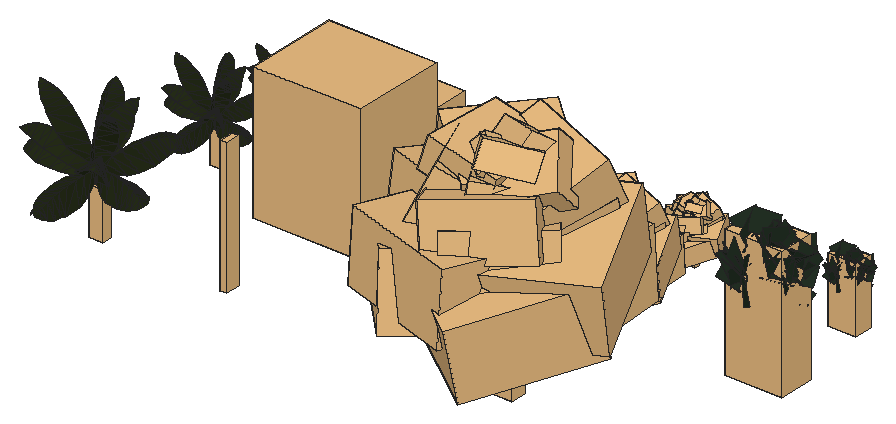
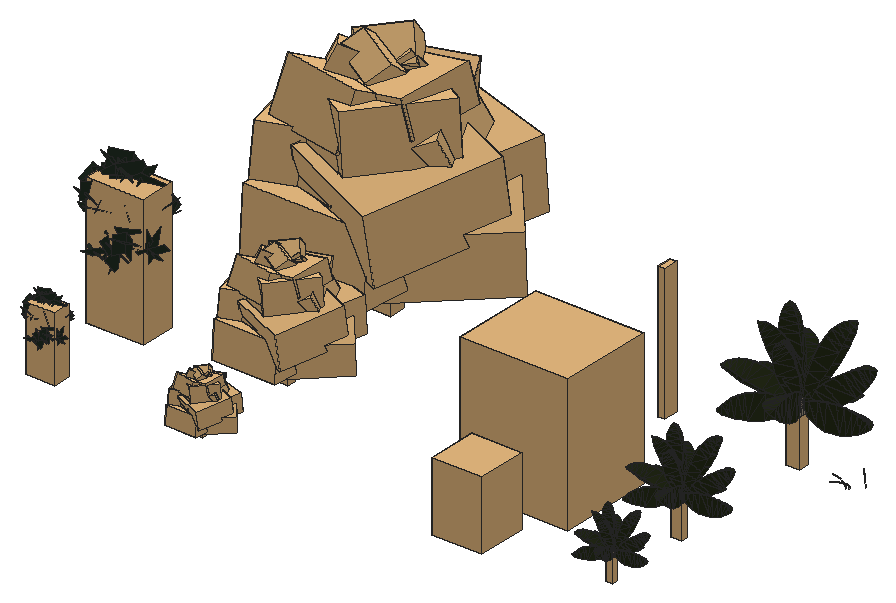
# SketchUp Ruby script. Lengths in inches.
U = 1.inch
M = Sketchup.active_model
def pt(a) = Geom::Point3d.new(a.map { |v| v * U })
def face(e, loops, mat)
  f = e.add_face(loops[0].map { |a| pt(a) })
  loops[1..].each { |l| e.add_face(l.map { |a| pt(a) }).erase! }
  f.material = f.back_material = mat if mat
  f
end
# faces: each face lists its corners as indices into pts; further lists are holes
def faces(e, pts, list, mat = nil) = list.each { |f| face(e, (f[0].is_a?(Array) ? f : [f]).map { |l| l.map { |i| pts[i] } }, mat) }
# xy, xz, yz: faces in a plane at the given z, y or x. An outline is a flat list of corners, or four numbers for a rectangle; further outlines are holes
def ring(l) = l.size == 4 ? [[l[0], l[1]], [l[2], l[1]], [l[2], l[3]], [l[0], l[3]]] : l.each_slice(2).to_a
def flat(e, list, mat, &to3) = list.each { |f| face(e, (f[0].is_a?(Array) ? f : [f]).map { |l| ring(l).map { |u, v| to3.(u, v) } }, mat) }
def xy(e, z, list, mat = nil) = flat(e, list, mat) { |x, y| [x, y, z] }
def xz(e, y, list, mat = nil) = flat(e, list, mat) { |x, z| [x, y, z] }
def yz(e, x, list, mat = nil) = flat(e, list, mat) { |y, z| [x, y, z] }
def lines(e, pts, list) = list.each { |a, b| e.add_line(pt(pts[a]), pt(pts[b])) }
# prism: a flat outline (further loops are holes) pulled along v
def prism(e, loops, v, mat = nil)
  f = face(e, loops, mat); d = Geom::Vector3d.new(v.map { |x| x * U })
  f.pushpull(f.normal.samedirection?(d) ? d.length : -d.length)
end
def box(e, o, s, mat = nil) = prism(e, [[o, [o[0] + s[0], o[1], o[2]], [o[0] + s[0], o[1] + s[1], o[2]], [o[0], o[1] + s[1], o[2]]]], [0, 0, s[2]], mat)
def at(x, y, z, deg = 0) = Geom::Transformation.translation(pt([x, y, z])) * Geom::Transformation.rotation(ORIGIN, Z_AXIS, deg.degrees)
def axes(o, x, y, z) = Geom::Transformation.new([*x, 0, *y, 0, *z, 0, *pt(o).to_a, 1])
def part(name) = M.definitions.add(name)
# library, detail: a bought-in or finely detailed component or shape, given as its bounding box
def library(name, o, s) = part(name).tap { |d| box(d.entities, o, s) }
def detail(e, o, s) = box(e.add_group.entities, o, s)
def put(e, d, t, mat = nil) = e.add_instance(d, t).tap { |i| i.material = mat if mat }
def group(e, t, mat = nil) = e.add_group.tap { |g| g.transformation = t; g.material = mat if mat }.entities
root = M.entities
M.materials.add("cocoanut_mat").color = [137, 122, 109]
M.materials.add("cocoanut_scrub").color = [165, 152, 134]
M.materials.add("coconut_test3_clean").color = [38, 45, 24]
M.materials.add("euc leaf02").color = [35, 48, 36]
c1 = library("Group\#110",[0,0,0],[259.75,161.77,589.29])
c2 = part("Blue Gum")
p = [[271.53,158.18,378.25],[270.5625,158.71,380.69],[270.37,158.83,381.17],[272.73,162.06,384.51],[213.85,150.08,152.75],[212.24,149.06,149.65],
  [150.49,110.24,344.32],[151.97,108.18,342.21],[217.47,152.58,206.91],[209.32,150.04,213.6],[153.27,112.37,338.72],[213.34,156.04,223.13],
  [212.17,155.27,219.89],[213.66,148.52,337.14],[212.6875,151.94,345.88],[201.33,160.36,0],[198.82,151.26,0.01],[228.58,150.59,468.55],
  [228.91,150.53,474.28],[226.95,148.99,472.86]]
faces(c2.entities,p,[[0,1,2],[1,0,3],[3,2,1]])
lines(c2.entities,p,[[4,5],[6,7],[8,9],[10,6],[7,10],[11,12],[13,14],[15,16],[17,18],[19,17],[18,19]])
put(c2.entities,c1,axes([324.42,234.92,0.08],[-1,0,-0.00067],[0,-1,0.00003],[-0.00067,0.00003,1]))
g1 = group(c2.entities,at(392.72,299.04,214.24))
p = [[-190.24,-45.24,49.75],[-155.8,-83.51,-0.1],[-171.1,-117.4,15.86],[-186.4,-151.3,31.82],[-220.85,-113.03,81.67],[-197.84,-62.08,57.68],
  [-156.97,-85.38,90],[-134.58,-101.98,23.98],[-207.62,-132.83,7.74],[-230.01,-116.24,73.77],[-175.11,-93.05,85.97],[-155.875,-47.35,89.82],
  [-171.875,-81.0625,28.63],[-175.09,-115.85,49.06],[-178.3125,-150.63,69.48],[-162.3125,-116.92,130.67],[-157.47,-64.63,99.96],[-108.86,-93.44,91.87],
  [-142.19,-103.1875,29.18],[-207.99,-128.51,68.93],[-174.66,-118.76,131.62],[-125.2,-99.73,101.74],[-105.25,-143.93,101.02],[-118.65,-122.91,33.83],
  [-139.46,-91.34,48.24],[-160.28,-59.76,62.65],[-146.87,-80.78,129.84],[-115.59,-128.24,108.18],[-69.65,-64.39,98.91],[-102.98,-74.13,36.22],
  [-135.88,-86.79,56.09],[-168.78,-99.45,75.97],[-135.45,-89.7,138.66],[-85.99,-70.68,108.78],[-206,0,112.1],[-205.51,-55.1,41.09],
  [-219.69,-93.37,71.26],[-233.87,-131.63,101.43],[-234.36,-76.53,172.4375],[-220.18,-38.26,142.27],[-213.05,-19.01,127.09],[-58.99,-92.56,99.73],
  [-109.77,-114.37,54.1],[-132.54,-82.69,64.86],[-155.3,-51.01,75.61],[-104.53,-29.2,121.24],[-70.31,-76.82,105.07],[-84.85,-14.67,104.44],
  [-93.72,-70.0625,59.84],[-130.5,-76.32,75.5],[-167.29,-82.57,91.16],[-158.42,-27.18,135.76],[-103.12,-17.78,112.22],[-170.99,-48.24,149.78],
  [-170.5,-103.34,78.77],[-268.88,-83.39,63.75],[-269.37,-28.29,134.76],[-195.43,-43.28,146.05],[-119.44,-162.62,158.17],[-165.08,-157.98,109.24],
  [-139.69,-139.86,87.75],[-114.31,-121.74,66.26],[-68.68,-126.38,115.19],[-94.0625,-144.5,136.68],[-106.83,-153.62,147.5],[-83.43,-178.22,123.11],
  [-129.0625,-173.58,74.18],[-150.32,-106.13,101.32],[-104.69,-110.78,150.25],[-88.71,-161.47,129.85],[-153.18,-33.52,154.23],[-187.55,-61.6,76.08],
  [-205.14,-103.18,99.27],[-222.72,-144.75,122.47],[-188.35,-116.67,200.62],[-170.77,-75.09,177.42],[-161.92,-54.17,165.75],[-126.95,-97.9375,165.85],
  [-161.32,-126.02,87.7],[-248.95,-80.33,110.85],[-214.58,-52.25,189],[-148.72,-86.59,171.6],[-365.27,-93.53,149.96],[-339.43,-156.16,87.91],
  [-290.4375,-139.67,92.34],[-241.45,-123.17,96.77],[-267.29,-60.54,158.83],[-340.93,-85.33,152.16],[-220,-209.94,88.83],[-192.18,-284.625,134.55],
  [-202.3,-275.33,156.35],[-232.93,-247.2,222.33],[-260.75,-172.52,176.61],[-240.375,-191.23,132.72],[-392.72,-100.24,198.19],[-366.88,-162.88,136.14],
  [-328.26,-131.57,121.3],[-289.64,-100.27,106.47],[-315.48,-37.63,168.52],[-373.54,-84.69,190.82],[-327.95,-161.62,221.67],[-317.1,-180.89,132.49],
  [-328.31,-131.57,120.9375],[-339.53,-82.25,109.39],[-350.38,-62.97,198.5625],[-333.52,-137.11,215.93],[-255.83,-236.76,152.47],[-329.61,-198.39,191.52],
  [-323.5,-175.58,181.2],[-305,-106.55,149.96],[-231.21,-144.93,110.9],[-243.52,-190.85,131.6875],[-205.5,-81.8,220.89],[-197.86,-85.86,131.43],
  [-243.5,-64.11,127],[-289.13,-42.35,122.57],[-296.77,-38.29,212.03],[-251.13,-60.04,216.46],[-228.17,-70.99,218.6875],[-234.33,-241.65,142.48],
  [-225.25,-222.09,231.79],[-228.94,-197.05,226.92],[-240.1,-121.29,212.17],[-249.18,-140.85,122.86],[-241.75,-191.25,132.67],[-227.68,-15.04,215.96],
  [-220.04,-19.1,126.5],[-266.95,-109.11,127.5],[-274.59,-105.04,216.95],[-239.33,-37.4,216.21],[-312.18,-35.14,201.88],[-307.82,-106.7,144.42],
  [-256.66,-99.36,139.9],[-205.5,-92.02,135.375],[-209.86,-20.46,192.83],[-286.77,-31.49,199.63],[-224.25,-107.3,143.78],[-158.47,-57.42,184.1],
  [-153.89,-76.52,200.79],[-140.05,-134.32,251.29],[-205.83,-184.2,210.96],[-215.04,-145.75,177.37],[-371.18,-63.42,218.95],[-318.87,-74.08,144.18],
  [-278.67,-86.3125,174.61],[-238.47,-98.55,205.04],[-290.78,-87.88,279.82],[-351.21,-69.49,234.07],[-314.82,-59.28,247.3],[-323.0625,-96.32,163.62],
  [-272.16,-89.61,156.15],[-221.26,-82.9,148.67],[-213.02,-45.87,232.35],[-289.54,-55.95,243.59],[-269.6,-260.65,169.64],[-261.02,-289.45,256.47],
  [-255.15,-265.53,264.0625],[-237.36,-193.15,287.04],[-245.94,-164.36,200.22],[-257.77,-212.5,184.93],[-219.98,-94.58,184.38],[-135.38,-92.14,220.14],
  [-132.93,-117.5625,216.66],[-125.5,-194.48,206.12],[-210.1,-196.92,170.36],[-242.72,-259.5,171.19],[-311.27,-292.91,222.44],[-317.8125,-269.04,229.65],
  [-337.62,-196.84,251.48],[-269.07,-163.43,200.23],[-255.89,-211.46,185.71],[-204.01,-188.2,177.79],[-188.33,-208.64,265.98],[-194.51,-184.59,272.89],
  [-213.23,-111.83,293.8125],[-228.92,-91.39,205.62],[-216.46,-139.79,191.7],[-111.12,-172.19,178.4],[-144.16,-223.61,247],[-146.96,-202.62,261.69],
  [-155.45,-139.1,306.14],[-122.41,-87.68,237.53],[-116.76,-129.9375,207.97],[-92.3,-219.25,321.53],[-140.07,-175.86,256.125],[-105.48,-191.84,220.91],
  [-70.89,-207.83,185.69],[-23.13,-251.22,251.1],[-75.12,-227.1875,304.03],[-95.32,-86.56,260.02],[-28.15,-67.53,258.27],[-24.95,-79.6,243.18],
  [-15.25,-116.11,197.51],[-82.42,-135.13,199.26],[-88.87,-110.84,229.64],[-230.35,-182.42,199.75],[-240.26,-200.67,289.25],[-235.09,-176.09,295.07],
  [-219.44,-101.74,312.67],[-209.53,-83.5,223.17],[-219.9375,-132.96,211.46],[-140.68,-151.65,266.01],[-78.24,-142.94,332.84],[-63.08,-129.17,317.2],
  [-17.2,-87.5,269.85],[-79.64,-96.22,203.02],[-110.16,-123.93,234.52],[-181.78,-155.46,254.29],[-197.87,-106.1875,330.15],[-215.8125,-92.48,317.72],
  [-270.1,-51.01,280.11],[-254.02,-100.28,204.25],[-217.9,-127.875,229.27],[-219.05,-237.83,228.68],[-246.19,-265.11,312.11],[-270.4375,-258.25,306.72],
  [-343.82,-237.49,290.4],[-316.68,-210.21,206.96],[-267.86,-224.02,217.82],[-221.64,-245.99,220.16],[-255.74,-296.14,289.1875],[-278.74,-284.87,286.3125],
  [-348.35,-250.78,277.61],[-314.25,-200.64,208.59],[-267.95,-223.32,214.37],[-214.08,-176.63,246.6],[-287.9,-162.75,299.5],[-289.8,-138.53,290.89],
  [-295.55,-65.24,264.85],[-221.72,-79.12,211.94],[-273.56,-277.41,225.52],[-332.72,-264.05,294.53],[-330.67,-238.52,291.65],[-324.47,-161.27,282.95],
  [-265.3,-174.62,213.93],[-269.43,-226.01,219.72],[-125.42,-280.5,273.74],[-154.49,-208.42,224.74],[-56.47,-175.26,217.08],[-27.39,-247.34,266.08],
  [-101.07,-272.26,271.84],[-137.08,-126.63,220.68],[-181.31,-63.4,270.55],[-159.07,-51.25,275.29],[-91.8,-14.51,289.63],[-47.57,-77.74,239.76],
  [-92.33,-102.1875,230.22],[-238.16,-243.49,222.62],[-218.34,-248.07,312.22],[-217.08,-222.36,313.49],[-213.28,-144.56,317.34],[-233.09,-139.97,227.74],
  [-235.625,-191.73,225.18],[-96.8,-128.7,236.99],[-25.62,-162.74,224.18],[-29.7,-177.8,240.28],[-42.05,-223.37,289.02],[-113.23,-189.33,301.82],
  [-105.01,-159.01,269.41],[-190.11,-164.1875,296.41],[-166.86,-101.93,340.84],[-154.3,-94.29,323.91],[-116.3,-71.16,272.67],[-139.55,-133.41,228.25],
  [-164.83,-148.8,262.33],[-190.89,-165.45,228.74],[-213.01,-227.55,273.96],[-199.51,-220.6,290.46],[-158.68,-199.56,340.39],[-136.56,-137.46,295.18],
  [-163.73,-151.45,261.96],[-108.84,-65.86,242.35],[-143.91,-74.96,326.78],[-145.22,-100.52,323.73],[-149.17,-177.86,314.51],[-114.09,-168.76,230.08],
  [-111.47,-117.3125,236.21],[-131.79,-76.12,256.875],[-89.01,-36.19,327.71],[-66.95,-47.86,321.26],[-0.2,-83.16,301.74],[-42.99,-123.09,230.91],
  [-87.39,-99.61,243.89],[-191.96,-179.86,282.46],[-135.02,-196.07,336.18],[-121.21,-181.46,326.24],[-79.42,-137.25,296.18],[-136.36,-121.05,242.47],
  [-164.16,-150.45,262.47],[-230.13,-253.21,246.97],[-260.13,-299.04,320.74],[-267.04,-276.89,331.97],[-287.96,-209.88,365.95],[-257.97,-164.06,292.17],
  [-244.05,-208.64,269.57],[-280.97,-237.22,246.96],[-334.39,-225.07,320.72],[-316.05,-210.87,331.95],[-260.54,-167.9,365.9375],[-207.12,-180.05,292.18],
  [-123.3,-254.01,336.04],[-125.12,-228.29,247.85],[-81.63,-201.01,255.39],[-38.14,-173.74,262.92],[-36.32,-199.46,351.11],[-101.69,-240.46,339.78],
  [-68.26,-134.5,260.14],[-26.24,-201.97,251.74],[-44.5,-214.15,256.34],[-99.74,-251,270.27],[-141.76,-183.53,278.67],[-121.3,-170.4,347.79],
  [-129.86,-181.96,257.04],[-33.4,-220.07,253.73],[-24.85,-208.51,344.48],[-97.34,-179.87,346.97],[-78.09,-121.04,341.08],[-129.1,-143.71,268.11],
  [-128.64,-193.18,283.74],[-128.18,-242.65,299.36],[-77.17,-219.98,372.34],[-77.86,-145.61,348.85],[-177.42,-71.46,329.51],[-152.53,-122.65,273.39],
  [-155.7,-156.33,303.27],[-158.88,-190.01,333.16],[-183.78,-138.82,389.27],[-179,-88.19,344.35],[-150.51,-90.39,274.04],[-160.0625,-83.41,365.16],
  [-137.04,-94.48,368.65],[-67.4,-127.95,379.21],[-57.85,-134.93,288.09],[-104.18,-112.66,281.07],[-94.02,-187.3,327.96],[-81.13,-138.55,389.98],
  [-69.09,-124.83,376.95],[-32.66,-83.33,337.53],[-45.54,-132.09,275.51],[-69.78,-159.69,301.74],[-118.35,-128.14,277.49],[-134.07,-116.2,367.22],
  [-118.18,-95.9,367.54],[-70.12,-34.49,368.49],[-54.4,-46.4375,278.76],[-86.375,-87.29,278.12],[-130.67,-185.64,278.8125],[-99.69,-223.89,341.79],
  [-81.85,-210.3,341.52],[-27.87,-169.2,340.6875],[-58.85,-130.95,277.71],[-94.76,-158.29,278.26],[-124.09,-168.51,302.87],[-98.25,-187.53,376.08],
  [-77.34,-181.72,370.43],[-14.08,-164.14,353.32],[-39.93,-145.12,280.11],[-82.01,-156.82,291.49],[-222.9,-199.13,376.1],[-220.07,-149.45,341.44],
  [-227.34,-168.57,313.98],[-234.62,-187.6875,286.52],[-237.45,-237.37,321.18],[-230.17,-218.25,348.64],[-226.51,-208.63,362.46],[-66.91,-203,314.13],
  [-2.98,-185.26,358.72],[-4.41,-163.74,352.56],[-8.73,-98.64,333.94],[-72.66,-116.39,289.35],[-169.41,-164.76,388.4],[-177.97,-176.3125,297.65],
  [-129.74,-195.37,296],[-81.52,-214.43,294.34],[-72.96,-202.87,385.09],[-145.46,-174.22,387.58],[-154.72,-129.21,384.88],[-129.15,-146.67,298.38],
  [-129.71,-197.46,308.96],[-130.27,-248.25,319.53],[-155.84,-230.78,406.04],[-155,-154.4375,390.14],[-202.43,-168.15,321.54],[-179.78,-204.63,388.96],
  [-158.3,-199.98,384.5],[-93.32,-185.9,371.01],[-115.96,-149.42,303.58],[-159.19,-158.79,312.5625],[-197.46,-225.01,341.1],[-194.63,-175.33,306.4375],
  [-260.05,-161.8125,321.53],[-262.88,-211.49,356.1875],[-213.71,-221.65,344.85],[-157.48,-194.21,341.46],[-113.86,-228.8,398.82],[-95.37,-218.73,391.1],
  [-39.42,-188.27,367.76],[-83.04,-153.67,310.41],[-120.26,-173.9375,325.9375],[-193.32,-187.43,311.78],[-211.98,-162.83,385.51],[-194.23,-149.13,385.64],
  [-140.53,-107.67,386.06],[-121.86,-132.27,312.33],[-157.59,-159.85,312.05],[-258.44,-158.87,437.95],[-244.84,-121.05,355.33],[-234.18,-168.04,336.09],
  [-223.52,-215.03,316.85],[-237.12,-252.84,399.47],[-253.15,-182.21,428.39],[-193.45,-225.28,404.25],[-172.56,-175.18,330.125],[-129.23,-203.0625,324.0625],
  [-85.9,-230.95,318],[-106.8,-281.05,392.12],[-171.93,-239.14,401.24],[-189.32,-183.99,368.07],[-165.25,-149.36,435.97],[-148.5625,-139.1,425.06],
  [-98.07,-108.05,392.03],[-122.15,-142.68,324.13],[-155.73,-163.33,346.1],[-155.65,-206.76,334.06],[-167.83,-218.04,412.25],[-167.96,-195.875,415.63],
  [-168.38,-128.8,425.86],[-156.21,-117.52,347.67],[-155.93,-162.14,340.86],[-145.4375,-206.81,336.52],[-133.41,-216.07,415],[-138.07,-194.41,418.47],
  [-152.15,-128.87,428.97],[-164.18,-119.61,350.49],[-154.81,-163.21,343.5],[-277.65,-112.64,443.48],[-209.06,-142.23,389.99],[-242.625,-172.43,364.44],
  [-276.2,-202.63,338.89],[-344.79,-173.04,392.38],[-294.33,-127.64,430.79],[-116.84,-180.91,416.6],[-166.69,-214.06,346.91],[-201.41,-176.24,354.36],
  [-236.13,-138.41,361.82],[-186.28,-105.26,431.51],[-134.09,-162.12,420.31],[-150.67,-209.23,358.7],[-156.56,-222.56,437.29],[-138.24,-210.16,440.97],
  [-82.8125,-172.64,452.1],[-76.93,-159.31,373.5],[-113.8,-184.27,366.1],[-154.14,-165.42,373.5],[-127.09,-136.44,442.91],[-107.04,-145.81,439.23],
  [-46.4,-174.14,428.11],[-73.46,-203.11,358.7],[-161.71,-108.91,440.68],[-158.5,-155.86,361.76],[-202.41,-180.14,374.96],[-246.32,-204.43,388.15],
  [-249.52,-157.48,467.07],[-183.52,-120.98,447.23]]
faces(g1,p,[[0,1,2,3,4,5],[6,7,2,8,9,10],[11,12,13,14,15,16],[17,18,13,19,20,21],[22,23,24,25,26,27],[28,29,30,31,32,33],[34,35,36,37,38,39,40],[41,42,43,44,45,46],
  [47,48,49,50,51,52],[53,54,36,55,56,39,57],[58,59,60,61,62,63,64],[65,66,60,67,68,63,69],[70,71,72,73,74,75,76],[77,78,72,79,80,75,81],[82,83,84,85,86,87],[88,89,90,91,92,93],
  [94,95,96,97,98,99],[100,101,102,103,104,105],[106,107,108,109,110,111],[112,113,114,115,116,117,118],[119,120,121,122,123,124],[125,126,114,127,128,117,129],[130,131,132,133,134,135],[136,137,138,139,140,141],
  [142,143,144,145,146,147],[148,149,150,151,152,153],[154,155,156,157,158,159],[160,161,162,163,164,141],[165,166,167,168,169,170],[171,172,173,174,175,176],[177,178,179,180,181,182],[183,184,185,186,187,188],
  [189,190,191,192,193,194],[195,196,197,198,199,200],[201,202,203,204,205,206],[207,208,209,210,211,212],[213,214,215,216,217,218],[219,220,221,222,223,224],[225,226,227,228,229,212],[230,231,232,233,234,235],
  [236,237,185,238,239,240],[241,242,243,244,245,246],[247,248,249,250,251,252],[253,254,255,256,257,258],[259,260,261,262,263,264],[265,266,267,268,269,270],[271,272,273,274,275,276],[277,278,279,280,281,282],
  [283,284,285,286,287,288],[289,290,291,292,293,294],[295,296,297,298,299,294],[300,301,302,303,304,305],[306,307,308,309,310,258],[311,312,302,313,314,315],[316,317,318,319,320,321],[322,323,324,325,326,327],
  [328,329,330,331,332,333],[334,335,336,337,338,339],[340,341,342,343,344,345],[346,347,348,349,350,351],[352,353,354,355,356,357],[358,359,360,361,362,363,364],[365,366,367,368,369,339],[370,371,372,373,374,375],
  [376,377,378,379,380,381],[382,383,384,385,386,387],[388,389,360,390,391,363,392],[393,394,395,396,397,398],[399,400,401,402,403,404],[405,406,407,408,409,410],[411,412,413,414,415,416],[417,418,419,420,421,422],
  [423,424,425,426,427,428],[429,430,431,432,433,434],[435,436,437,438,439,440],[441,442,443,444,445,446],[447,448,449,450,451,452],[453,454,455,456,457,452],[458,459,460,461,462,463]],"euc leaf02")
c3 = library("Small Tree",[-46.3125,-47.83,0],[89.1875,89.28,122.02])
c4 = part("coconut_half")
p = [[54.48,2.6,2.17],[90.24,0,0],[105.09,35.75,42.48],[115.87,5,0],[128.48,35.75,36.0625],[152.37,21,0],
  [152.37,35.75,27.13],[169.19,35.75,17.77],[57.93,35.75,46.59],[42.36,5.25,5.16],[79.93,35.75,46.59],[41.85,35.75,44.23],
  [28.04,8.5,7.49],[27.85,35.75,39.58],[16.59,14.5,9.63],[9.27,35.75,26.98],[6.26,23.5,11.78],[16.71,35.75,32.89],
  [0,35.75,14.25]]
faces(c4.entities,p,[[0,1,2],[1,3,4],[1,4,2],[3,5,6],[3,6,4],[5,7,6],[0,8,9],[0,10,8],
  [0,2,10],[9,11,12],[9,8,11],[12,13,14],[12,11,13],[14,15,16],[14,17,15],[14,13,17],
  [18,16,15]],"coconut_test3_clean")
c5 = part("Group\#14")
put(c5.entities,c4,at(0,0,0))
put(c5.entities,c4,axes([0,71.5,0],[1,0,0],[0,-1,0],[0,0,1]))
c6 = part("coconut3_top")
put(c6.entities,c5,axes([-176.42,-40.5625,245.57],[1,0,0],[0,0.96593,-0.25882],[0,0.25882,0.96593]))
g2 = group(c6.entities,at(-4.7,-151.6,178.32))
put(g2,c4,axes([0,0,0],[0.14944,0.9543,0.25882],[-0.87562,0.00613,0.48296],[0.4593,-0.2988,0.83652]))
put(g2,c4,axes([-62.61,0.4375,34.53],[0.14944,0.9543,0.25882],[0.87562,-0.00613,-0.48296],[0.4593,-0.2988,0.83652]))
put(c6.entities,c5,axes([171.02,-15.64,245.06],[-0.94665,0.32227,0],[-0.31128,-0.91439,-0.25882],[-0.08341,-0.24501,0.96593]))
put(c6.entities,c5,axes([41.29,183.8,264.73],[-0.39574,-0.90582,-0.15126],[0.91636,-0.40035,0],[-0.06056,-0.13861,0.98849]))
put(c6.entities,c5,axes([-77.19,156.92,280.49],[0.30009,-0.91813,-0.25882],[0.86338,0.14605,0.48296],[-0.40562,-0.36839,0.83652]))
put(c6.entities,c5,axes([-112.56,-104.35,340.4],[0.76036,0.41456,-0.5],[-0.63406,0.64068,-0.43301],[0.14083,0.64627,0.75]))
put(c6.entities,c5,axes([119.49,-113.07,311.83],[-0.54618,0.67208,-0.5],[-0.83762,-0.43208,0.3342],[0.00857,0.60135,0.79894]))
put(c6.entities,c5,axes([103.27,116.54,337.13],[-0.75167,-0.49748,-0.43301],[0.65951,-0.56129,-0.5],[0.0057,-0.66141,0.75]))
put(c6.entities,c5,axes([-111.91,-75.47,434.48],[0.55528,0.30275,-1.09544],[-0.10884,0.68367,0.13377],[0.95166,0.05419,0.49738]))
put(c6.entities,c5,axes([96.22,-37.8,421.8],[-0.43628,0.34579,-0.96422],[-0.35338,-0.74638,-0.10777],[-0.75439,0.29273,0.44631]))
put(c6.entities,c5,axes([-41.59,80.66,420.02],[0.06101,-0.43197,-0.99256],[0.722,0.18761,-0.03727],[0.23024,-0.81295,0.36796]))
put(c6.entities,c5,axes([62.57,69.42,421.8],[-0.49424,-0.25619,-0.96422],[0.53593,-0.62829,-0.10777],[-0.57624,-0.5681,0.44631]))
c7 = part("cocoanut_mat")
yz(c7.entities,2,[[0.45,5,4.17,5,4.55,7.22,0,7.22]],"cocoanut_mat")
p = [[1.5,0.95,2.55],[0,1.26,0],[1.5,4.17,2.55],[0,3.01,0.06],[2,0.45,5],[2,4.17,5],
  [1.5,4.82,10.82],[1.5,0,9.97],[2,4.55,7.22],[2,0,7.22],[1,0.99,11.1],[1,3.98,11.36]]
faces(c7.entities,p,[[0,1,2],[3,2,1],[4,0,2,5],[6,7,8],[9,8,7],[7,6,10],[11,10,6]],"cocoanut_mat")
c8 = part("Coconut Palm")
xy(c8.entities,112.14,[[122.28,106.09,125.08,107.25,126.24,110.05,125.08,112.85,122.28,114.01,119.48,112.85,118.32,110.05,119.48,107.25]])
detail(c8.entities,[118.32,101.24,0],[25.61,17.45,83.17])
put(c8.entities,c6,axes([125.26,110.5,-76.06],[0.71,0,0],[0,0.71,0],[0,0,0.71]))
g3 = group(c8.entities,at(117.6,103.69,82.125))
p = [[4.68,2.4,1.05],[4.68,2.4,30.02],[1.88,3.56,30.02],[1.88,3.56,1.05],[7.48,3.56,1.05],[7.48,3.56,30.02],
  [0.72,6.36,30.02],[0.72,6.36,1.05],[8.64,6.36,1.05],[8.64,6.36,30.02],[1.88,9.16,30.02],[1.88,9.16,1.05],
  [7.48,9.16,1.05],[7.48,9.16,30.02],[4.68,10.32,30.02],[4.68,10.32,1.05]]
faces(g3,p,[[0,1,2,3],[4,5,1,0],[2,6,7,3],[4,8,9,5],[6,10,11,7],[8,12,13,9],[11,10,14,15],[15,14,13,12]],"cocoanut_scrub")
put(g3,c7,axes([8.73,9,14.81],[0.95137,0.17914,0.2506],[-0.24236,0.93742,0.25],[-0.19013,-0.29858,0.93525]))
put(g3,c7,axes([1.89,13.92,14.26],[-0.95388,0.23795,0.18301],[-0.27087,-0.94506,-0.18301],[0.17341,-0.30035,1.29434]))
put(g3,c7,axes([3.98,0.08,4.09],[0.521,-0.82169,0.23104],[0.85353,0.50368,-0.13339],[-0.00676,0.2667,0.96376]))
put(g3,c7,axes([2.8,2.4,6.76],[-0.16755,-0.98247,0.08171],[0.984,-0.16156,0.07513],[-0.09879,0.15157,1.61993]))
put(g3,c7,axes([8.29,10.47,4.97],[0.02489,0.99575,0.08868],[-0.99708,0.03112,-0.06968],[-0.11254,-0.13523,1.55005]))
put(g3,c7,axes([10.54,2.88,6.76],[0.95137,0.17914,0.2506],[-0.115,0.96125,-0.25056],[-0.28577,0.20956,0.9351]))
c9 = library("trunk\#1",[0,0,0],[11.46,27.17,238.43])
c10 = library("Group\#113",[-22.47,-14.25,0],[191.27,167.9,240.05])
c11 = library("Pine branch",[-164.19,86.97,62.64],[148.2,83.79,137.08])
c12 = part("Gruppe\#2")
detail(c12.entities,[0.71,-7.7,0],[22.57,19.31,263.85])
c13 = part("Kiefer Pine")
put(c13.entities,c11,axes([141.72,46.52,161.66],[-0.02916,-0.63772,0.00271],[0.15221,-0.00358,0.48358],[-0.6193,0.02915,0.11872]))
put(c13.entities,c11,axes([97.98,30.67,99.84],[-0.47537,-0.59297,0.00413],[0.14389,-0.11021,0.73807],[-0.57526,0.46243,0.1812]))
put(c13.entities,c11,axes([147.43,170.77,85.84],[0.66331,0.36209,0.08066],[-0.16152,0.13314,0.73061],[0.33395,-0.6548,0.19316]))
put(c13.entities,c11,axes([126.12,172.51,50.8],[0.58404,0.48629,0.00413],[-0.11903,0.13668,0.73807],[0.47151,-0.56784,0.1812]))
put(c13.entities,c11,axes([129.28,102.66,199.18],[0.3329,0.20176,-0.07756],[-0.04952,0.23763,0.27741],[0.2165,-0.24552,0.14305]))
put(c13.entities,c11,axes([28.39,91.46,58.6],[-0.71464,0.25212,0.05767],[-0.01186,-0.20123,0.73278],[0.25836,0.68814,0.19316]))
put(c13.entities,c11,axes([152.74,49.28,68.93],[0.33164,-0.67512,0.10878],[0.24998,0.23222,0.67911],[-0.63649,-0.26056,0.32339]))
put(c13.entities,c11,axes([-6.13,166.4,41.09],[-0.38774,0.8952,0.21972],[0.05521,-0.21538,0.97497],[0.92011,0.39016,0.03409]))
put(c13.entities,c11,axes([103.12,114.79,195.58],[-0.35402,0.16187,-0.07756],[-0.18541,-0.24864,0.1992],[0.04135,0.27092,0.22915]))
put(c13.entities,c11,axes([201.4375,150.2,7.87],[0.95266,-0.30403,0],[0.02078,0.06511,0.99766],[-0.30332,-0.95043,0.06835]))
put(c13.entities,c11,axes([149.14,-15.51,56.65],[-0.38076,-0.9108,0.15959],[0.00531,0.17044,0.98535],[-0.92466,0.37603,-0.06006]))
put(c13.entities,c11,axes([123.6,85.97,205.1],[0.23507,-0.19426,-0.06076],[0.16806,0.10538,0.1906],[-0.12474,-0.2241,0.1423]))
put(c13.entities,c11,axes([121.72,132.51,172.5],[0.36293,0.20783,-0.0399],[0.00027,0.10027,0.31921],[0.21403,-0.35254,0.06727]))
put(c13.entities,c11,axes([57.2,144.19,196.7],[-0.28797,0.37098,0.1914],[-0.03125,-0.30847,0.33516],[0.44369,0.21905,0.14782]))
put(c13.entities,c11,axes([93.55,232.34,18.61],[0.58552,0.78879,0.18704],[-0.06218,-0.18635,0.98051],[0.80827,-0.58574,-0.06006]))
put(c13.entities,c11,axes([33.34,105.32,91.71],[-0.72171,0.22385,0.08143],[-0.02606,-0.33247,0.68293],[0.23677,0.64572,0.32339]))
put(c13.entities,c11,axes([227.44,74.67,9.76],[0.6363,-0.72678,0.25867],[-0.14373,0.21775,0.96536],[-0.75793,-0.65144,0.03409]))
put(c13.entities,c11,axes([24.14,28.375,-27.51],[-1,0,0],[0,-0.06835,0.99766],[0,0.99766,0.06835]))
put(c13.entities,c12,at(97.66,98.27,0))
put(root,c2,axes([631.21,887.07,-58.68],[0.23912,0,0],[0,0.23912,0],[0,0,0.23912]))
put(root,c2,axes([653.69,1016.34,-58.6875],[0.11956,0,0],[0,0.11956,0],[0,0,0.11956]))
put(root,c3,axes([227.27,1020.97,-58.64],[0.61,0,0],[0,0.61,0],[0,0,0.61]))
put(root,c8,axes([7.66,693.22,-58.64],[0.61,0,0],[0,0.61,0],[0,0,0.61]))
put(root,c8,axes([31.1875,872.72,-58.64],[0.427,0,0],[0,0.427,0],[0,0,0.427]))
put(root,c8,axes([46.5,981.69,-58.64],[0.29463,0,0],[0,0.29463,0],[0,0,0.29463]))
put(root,c9,axes([223.87,751.96,-58.64],[0.61,0,0],[0,0.61,0],[0,0,0.61]))
put(root,c10,axes([181.45,875.65,-58.64],[0.61,0,0],[0,0.61,0],[0,0,0.61]))
put(root,c13,axes([424.73,674.11,-58.64],[0.915,0,0],[0,0.915,0],[0,0,0.915]))
put(root,c13,axes([462.46,871.97,-58.64],[0.4575,0,0],[0,0.4575,0],[0,0,0.4575]))
put(root,c13,axes([484.85,1012.1,-58.64],[0.22875,0,0],[0,0.22875,0],[0,0,0.22875]))
g4 = group(root,at(29.4,766.43,-58.625))
p = [[12.67,-0.07,9.36],[14.59,-0.08,9.61],[12.73,-0.07,9.31],[10.95,-0.0625,8.89],[9.24,-0.05,8.37],[7.64,-0.04,7.74],
  [6.15,-0.03,7.02],[4.81,-0.03,6.2],[3.62,-0.02,5.3],[2.59,-0.01,4.34],[1.74,-0.01,3.3125],[1.07,-0.01,2.24],
  [0.6,0,1.13],[0.33,0,0],[0,0,0],[0.22,0,1.16],[0.66,0,2.3],[1.32,-0.01,3.39],
  [2.17,-0.01,4.44],[3.22,-0.02,5.43],[4.45,-0.02,6.34],[5.85,-0.03,7.15],[7.38,-0.04,7.875],[9.05,-0.05,8.49],
  [10.82,-0.0625,8.98]]
faces(g4,p,[[0,1,2,3,4,5,6,7,8,9,10,11,12,13,14,15,16,17,18,19,20,21,22,23,24]])
g5 = group(root,at(27,764.18,-58.625))
p = [[0.46,0.39,0],[0.2,0.17,0],[0,0,0.91],[0.08,0.07,1.82],[0.45,0.38,2.72],[1.1,0.93,3.57],
  [2,1.7,4.37],[3.15,2.68,5.08],[4.5,3.83,5.69],[6.03,5.13,6.19],[7.7,6.55,6.57],[9.47,8.05,6.81],
  [11.29,9.6,6.91],[13.11,11.15,6.86],[11.32,9.63,6.87],[9.55,8.12,6.74],[7.83,6.66,6.48],[6.21,5.28,6.09],
  [4.73,4.02,5.59],[3.42,2.91,4.98],[2.31,1.96,4.28],[1.42,1.21,3.5],[0.78,0.67,2.66],[0.41,0.35,1.79],
  [0.3,0.25,0.89]]
faces(g5,p,[[0,1,2,3,4,5,6,7,8,9,10,11,12,13,14,15,16,17,18,19,20,21,22,23,24]])
g6 = group(root,at(17.89,754.59,-58.625))
p = [[8.91,-9.01,9.36],[10.26,-10.37,9.61],[8.95,-9.05,9.31],[7.7,-7.78,8.89],[6.5,-6.57,8.37],[5.37,-5.43,7.74],
  [4.33,-4.375,7.02],[3.38,-3.42,6.2],[2.54,-2.57,5.3],[1.82,-1.84,4.34],[1.22,-1.24,3.3125],[0.75,-0.76,2.24],
  [0.42,-0.43,1.13],[0.23,-0.23,0],[0,0,0],[0.16,-0.16,1.16],[0.47,-0.47,2.3],[0.93,-0.9375,3.39],
  [1.53,-1.55,4.44],[2.27,-2.29,5.43],[3.13,-3.17,6.34],[4.11,-4.16,7.15],[5.19,-5.25,7.875],[6.36,-6.44,8.49],
  [7.61,-7.69,8.98]]
faces(g6,p,[[0,1,2,3,4,5,6,7,8,9,10,11,12,13,14,15,16,17,18,19,20,21,22,23,24]])
